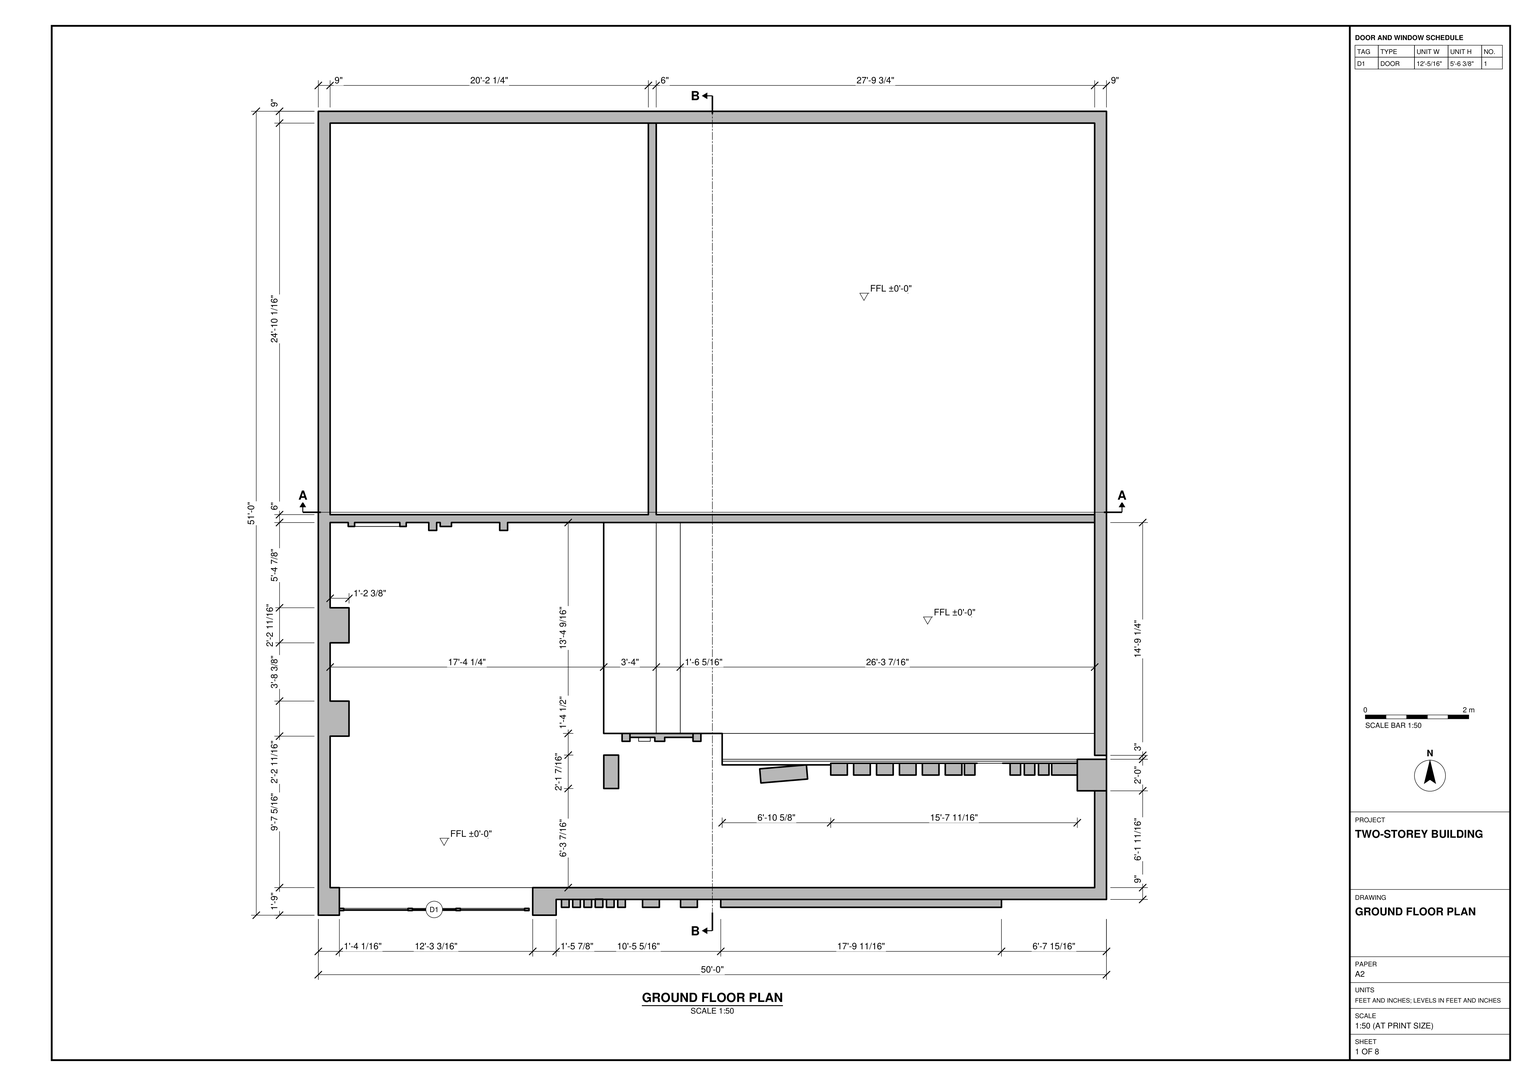
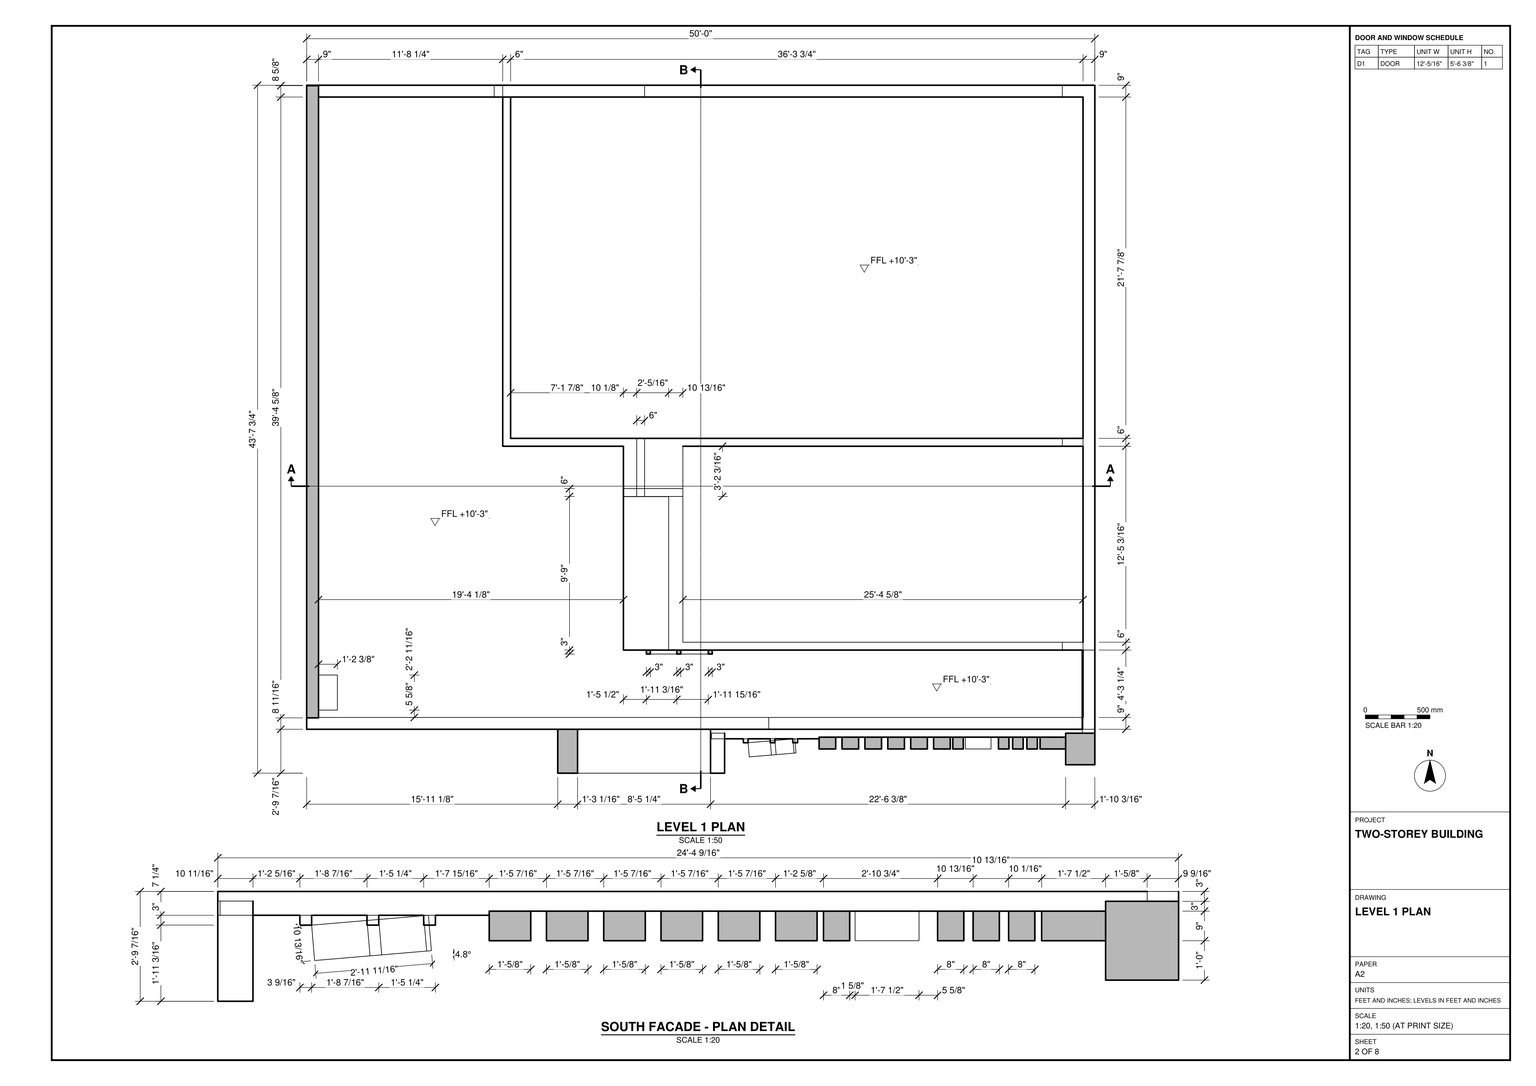
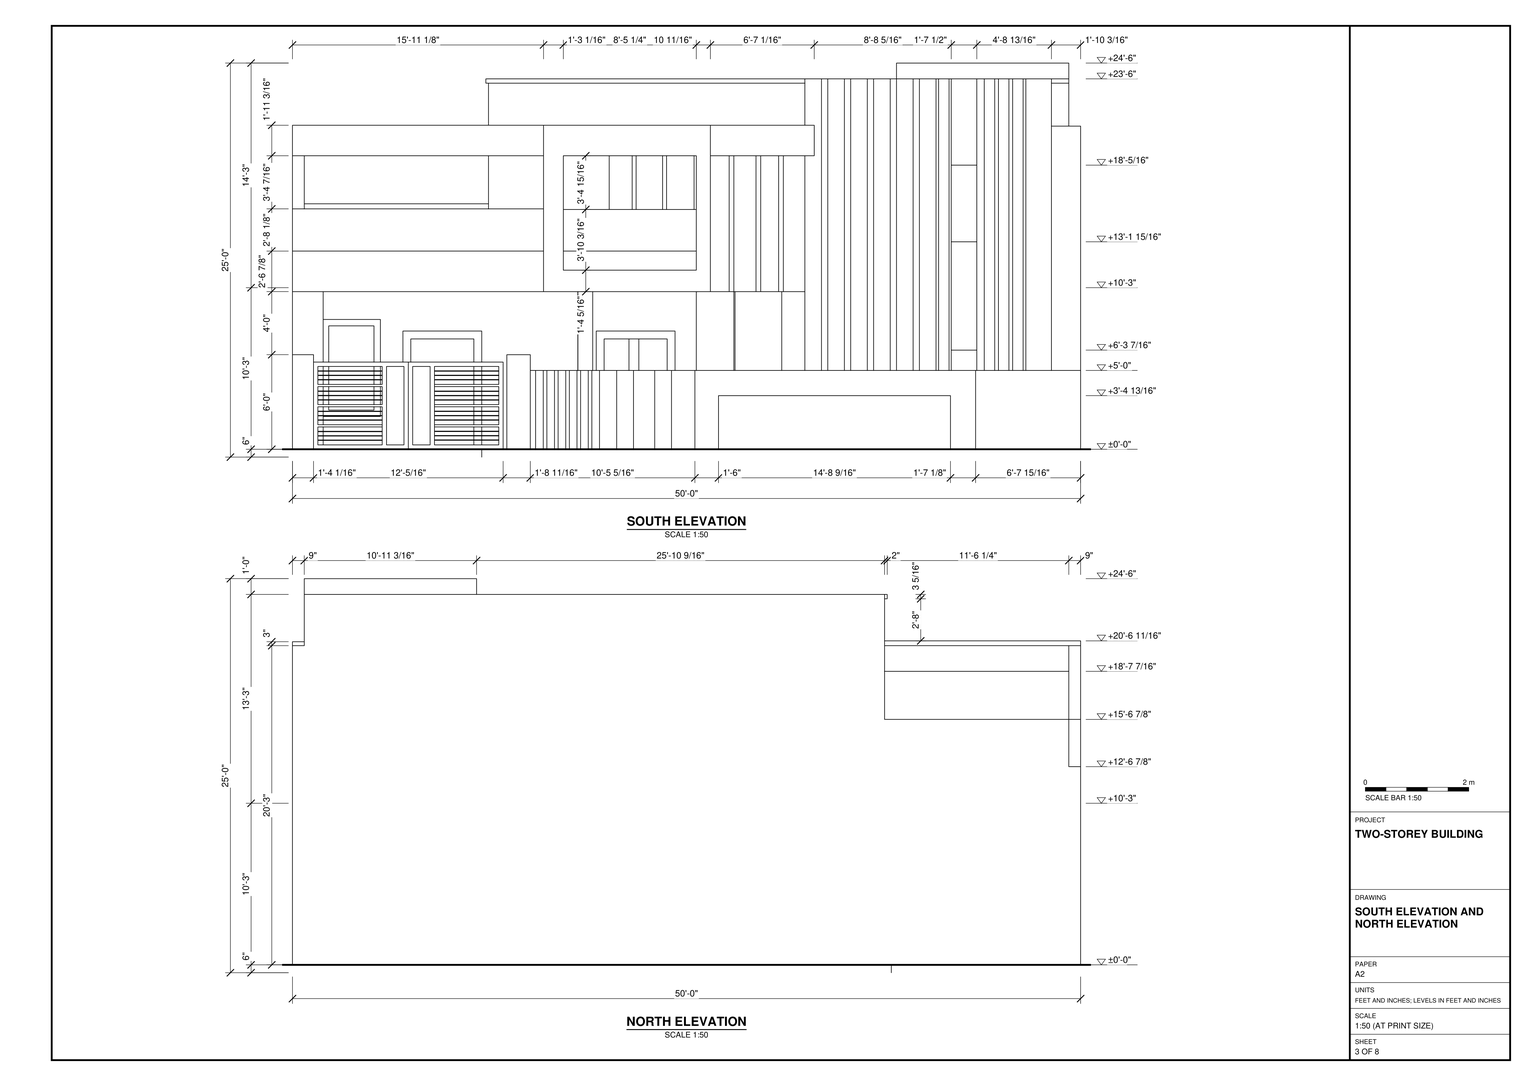
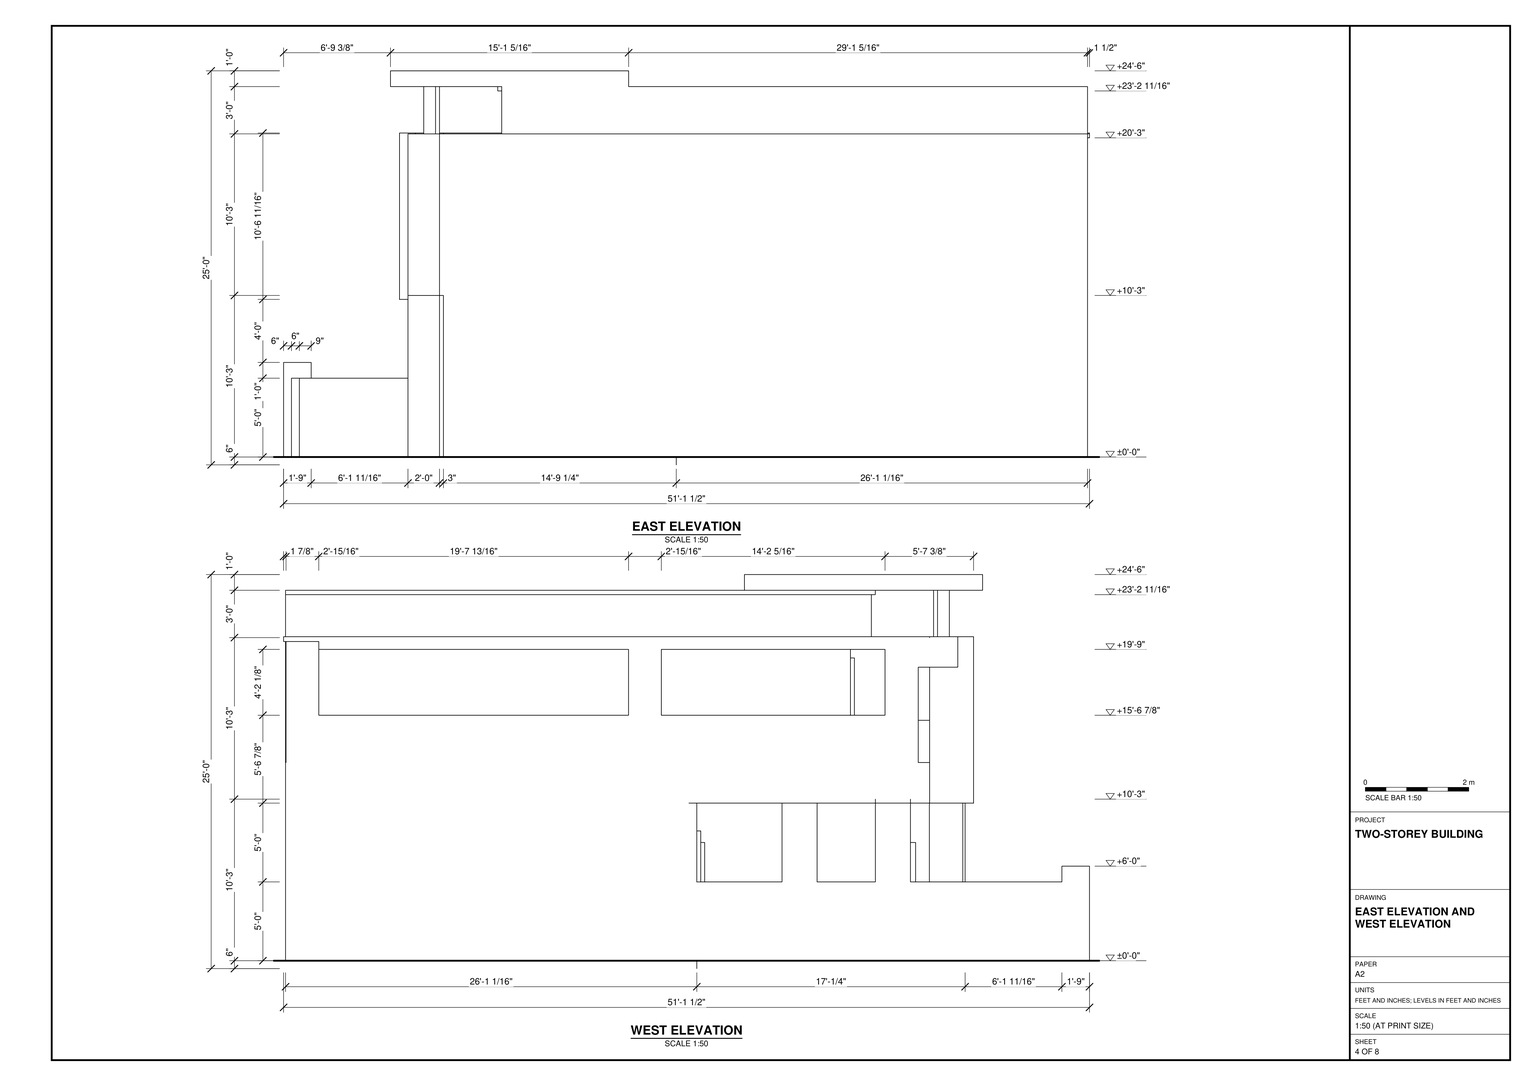
Build the two-storey building in SketchUp using task_files/diagram_01.pdf. Work in feet and inches. Set the overall width to 50'-0", the overall depth to 51'-1 1/2", and the overall height to 24'-6". Use ±0'-0" for the ground floor and +10'-3" for the upper floor.

Lay out each floor from its own plan. Use the 9" perimeter walls and 6" partitions where dimensioned. On the ground floor, divide the rear portion into two unequal bays and retain the open space behind the front gate. On the upper floor, follow the offsets in the partition layout rather than copying the walls below. Model the floor slabs, flat roof sections and changes in roof height to match the sections and elevations.

Place the slatted gate between posts at the left of the south frontage. Use the south elevation for the framed openings and horizontal bands, and the façade plan detail for the spacing and projection of the tall vertical fins on the right. Include the rectangular panel in the low front wall. Keep walls, slabs and roof sections in separate groups or components, group each furniture or joinery piece separately, and use components for repeated parts. Any decor or loose items shown may be represented by suitable library components. Save one SketchUp model as output_files/two_storey_building_with_screened_south_facade.skp.

# SketchUp Ruby script. Lengths in inches.
U = 1.inch
M = Sketchup.active_model
def pt(a) = Geom::Point3d.new(a.map { |v| v * U })
def face(e, loops, mat)
  f = e.add_face(loops[0].map { |a| pt(a) })
  loops[1..].each { |l| e.add_face(l.map { |a| pt(a) }).erase! }
  f.material = f.back_material = mat if mat
  f
end
# faces: each face lists its corners as indices into pts; further lists are holes
def faces(e, pts, list, mat = nil) = list.each { |f| face(e, (f[0].is_a?(Array) ? f : [f]).map { |l| l.map { |i| pts[i] } }, mat) }
# xy, xz, yz: faces in a plane at the given z, y or x. An outline is a flat list of corners, or four numbers for a rectangle; further outlines are holes
def ring(l) = l.size == 4 ? [[l[0], l[1]], [l[2], l[1]], [l[2], l[3]], [l[0], l[3]]] : l.each_slice(2).to_a
def flat(e, list, mat, &to3) = list.each { |f| face(e, (f[0].is_a?(Array) ? f : [f]).map { |l| ring(l).map { |u, v| to3.(u, v) } }, mat) }
def xy(e, z, list, mat = nil) = flat(e, list, mat) { |x, y| [x, y, z] }
def xz(e, y, list, mat = nil) = flat(e, list, mat) { |x, z| [x, y, z] }
def yz(e, x, list, mat = nil) = flat(e, list, mat) { |y, z| [x, y, z] }
def lines(e, pts, list) = list.each { |a, b| e.add_line(pt(pts[a]), pt(pts[b])) }
# prism: a flat outline (further loops are holes) pulled along v
def prism(e, loops, v, mat = nil)
  f = face(e, loops, mat); d = Geom::Vector3d.new(v.map { |x| x * U })
  f.pushpull(f.normal.samedirection?(d) ? d.length : -d.length)
end
def box(e, o, s, mat = nil) = prism(e, [[o, [o[0] + s[0], o[1], o[2]], [o[0] + s[0], o[1] + s[1], o[2]], [o[0], o[1] + s[1], o[2]]]], [0, 0, s[2]], mat)
def at(x, y, z, deg = 0) = Geom::Transformation.translation(pt([x, y, z])) * Geom::Transformation.rotation(ORIGIN, Z_AXIS, deg.degrees)
def axes(o, x, y, z) = Geom::Transformation.new([*x, 0, *y, 0, *z, 0, *pt(o).to_a, 1])
def part(name) = M.definitions.add(name)
# library, detail: a bought-in or finely detailed component or shape, given as its bounding box
def library(name, o, s) = part(name).tap { |d| box(d.entities, o, s) }
def detail(e, o, s) = box(e.add_group.entities, o, s)
def put(e, d, t, mat = nil) = e.add_instance(d, t).tap { |i| i.material = mat if mat }
def group(e, t, mat = nil) = e.add_group.tap { |g| g.transformation = t; g.material = mat if mat }.entities
root = M.entities
M.materials.add("[0035_Tan]").color = [155, 133, 103]
M.materials.add("[0042_Sienna]").color = [145, 74, 40]
M.materials.add("[0042_Sienna]1").color = [160, 82, 45]
M.materials.add("[0135_DarkGray]").color = [81, 81, 81]
M.materials.add("[Color C08]").color = [63, 31, 0]
M.materials.add("[Color C08]1").color = [61, 30, 0]
M.materials.add("[Formica Graystone]").color = [149, 146, 135]
M.materials.add("[Granite Brown]").color = [81, 67, 58]
M.materials.add("[Granite Dark Gray]").color = [69, 68, 68]
M.materials.add("[Sandstone]").color = [118, 81, 52]
M.materials.add("[Tile Mosaic Multi]").color = [135, 103, 96]
M.materials.add("[Translucent Glass Blue]").color = [100, 149, 237]
M.materials["[Translucent Glass Blue]"].alpha = 0.5
M.materials.add("[Wood Square Tile 01]").color = [164, 91, 44]
M.materials.add("[Wood Veneer 01]").color = [120, 70, 37]
c1 = library("gate (1)",[0,0,0],[171.26,1.97,78.74])
xy(root,0,[[0,0,16.04,12],[163.22,0,181.0625,12],[185.11,6,190.93,12],[193.67,6,199.49,12],[202.24,6,208.05,12],
  [210.8,6,216.61,12],[219.36,6,225.18,12],[227.92,6,233.74,12],[246.83,6,259.625,12],[275.77,6,288.5625,12],
  [0,12,0,136.3,9,136.3,9,21,16.04,21,16.04,12],[163.22,12,163.22,21,591,21,591,12,216.61,12,216.61,12.25,210.8,12.25,210.8,12],[210.8,12,216.61,12.25],[591,12,600,94.6875],[577.78,94.6875,591,118.6875],
  [591,94.6875,600,118.6875],[217.33,96.45,228.58,121.89],[390.09,106.6875,402.74,115.6875],[407.52,106.6875,420.18,115.6875],[424.96,106.6875,437.61,115.6875],
  [442.4,106.6875,455.05,115.6875],[459.84,106.6875,472.49,115.6875],[477.27,106.6875,489.93,115.6875],[491.875,106.6875,499.86,115.6875],[526.625,106.6875,534.61,115.6875],
  [537.4375,106.6875,545.42,115.6875],[548.25,106.6875,556.23,115.6875],[558.31,106.6875,577.78,115.6875],[307.4375,114.4375,390.09,114.4375,390.09,115.6875,577.78,115.6875,577.78,117.25,307.4375,117.25],[307.4375,117.25,577.78,118.6875],
  [307.4375,118.6875,600,118.6875,600,121.6875,591,121.6875,591,138.375,307.4375,138.375],[591,121.6875,591,603,9,603,9,304.9375,251.25,304.9375,251.25,603,257.25,603,257.25,304.9375,591,304.9375,591,298.9375,0,298.9375,0,612,600,612,600,121.6875],[231.25,132.375,237.25,138.375],[256.18,132.375,257.25,132.375,257.25,138.375,237.25,138.375,237.25,135.375,256.18,135.375],[257.25,132.375,263.69,132.375,263.69,135.375,275.5625,135.375,275.5625,138.375,257.25,138.375],
  [285.25,132.375,291.25,138.375],[275.5625,135.375,285.25,138.375],[0,136.3,23.375,162.99],[217.25,138.375,257.25,298.9375],[257.25,138.375,275.5625,298.9375],
  [275.5625,138.375,591,298.9375],[0,162.99,9,207.36],[0,207.36,23.375,234.05],[0,234.05,9,298.9375],[84.1,292.9375,90.1,298.9375],
  [138.1,292.9375,144.1,298.9375],[9,304.9375,251.25,603],[257.25,304.9375,591,603]])
xy(root,0,[[306.36,6,324.34,12],[500.93,6,520.07,12]],"[0135_DarkGray]")
xy(root,0,[[[9,21,591,21,591,94.6875,577.78,94.6875,577.78,106.6875,558.31,106.6875,558.31,115.6875,556.23,115.6875,556.23,106.6875,548.25,106.6875,548.25,115.6875,545.42,115.6875,545.42,106.6875,537.4375,106.6875,537.4375,115.6875,534.61,115.6875,534.61,106.6875,526.625,106.6875,526.625,115.6875,499.86,115.6875,499.86,106.6875,491.875,106.6875,491.875,115.6875,489.93,115.6875,489.93,106.6875,477.27,106.6875,477.27,115.6875,472.49,115.6875,472.49,106.6875,459.84,106.6875,459.84,115.6875,455.05,115.6875,455.05,106.6875,442.4,106.6875,442.4,115.6875,437.61,115.6875,437.61,106.6875,424.96,106.6875,424.96,115.6875,420.18,115.6875,420.18,106.6875,407.52,106.6875,407.52,115.6875,402.74,115.6875,402.74,106.6875,390.09,106.6875,390.09,114.4375,307.4375,114.4375,307.4375,138.375,291.25,138.375,291.25,132.375,285.25,132.375,285.25,135.375,263.69,135.375,263.69,132.375,256.18,132.375,256.18,135.375,237.25,135.375,237.25,132.375,231.25,132.375,231.25,138.375,217.25,138.375,217.25,298.9375,144.1,298.9375,144.1,292.9375,138.1,292.9375,138.1,298.9375,90.1,298.9375,90.1,292.9375,84.1,292.9375,84.1,298.9375,9,298.9375,9,234.05,23.375,234.05,23.375,207.36,9,207.36,9,162.99,23.375,162.99,23.375,136.3,9,136.3],[217.33,96.45,228.58,121.89]]],"[Wood Square Tile 01]")
xy(root,16.24,[[336.92,100.66,336.01,111.4375,371.57,114.4375,372.48,103.66]])
xy(root,24.96,[[22.76,295.9375,66.9375,298.9375]],"[Granite Dark Gray]")
xy(root,29.83,[[27.63,295.9375,62.07,298.9375]],"[Granite Dark Gray]")
xy(root,40.81,[[324.34,6,500.93,12]],"[0135_DarkGray]")
xy(root,60,[[181.0625,12,210.8,12,210.8,12.25,216.61,12.25,216.61,12,600,12,600,94.6875,591,94.6875,591,21,181.0625,21],[210.8,12,216.61,12.25],[0,21,9,136.3],[0,162.99,9,207.36],[0,234.05,9,298.9375]])
xy(root,60,[[185.11,6,190.93,12],[193.67,6,199.49,12],[202.24,6,208.05,12],[210.8,6,216.61,12],[219.36,6,225.18,12],
  [227.92,6,233.74,12]],"[0042_Sienna]1")
xy(root,60,[[246.83,6,259.625,12],[275.77,6,288.5625,12],[306.36,6,520.07,12]],"[0135_DarkGray]")
xy(root,72,[[0,0,16.04,21],[163.22,0,181.0625,21]])
xy(root,75.46,[[501.49,106.6875,520.97,115.6875]])
xy(root,84,[[256.18,132.375,256.18,135.375,237.25,135.375,237.25,138.375,285.25,138.375,285.25,135.375,263.69,135.375,263.69,132.375]])
xy(root,84,[[237.25,132.375,256.18,135.375],[263.69,132.375,285.25,135.375],[90.1,292.9375,138.1,298.9375]],"[Sandstone]")
xy(root,90,[[231.25,132.375,291.25,138.375],[84.1,292.9375,144.1,298.9375]],"[Sandstone]")
xy(root,93.95,[[27.63,295.9375,62.07,298.9375]],"[Granite Dark Gray]")
xy(root,98.82,[[22.76,295.9375,66.9375,298.9375]],"[Granite Dark Gray]")
xy(root,120,[[332.4375,111.4375,336.01,114.4375],[336.01,111.4375,336.01,114.4375,352.875,114.4375,352.875,112.86],[352.875,111.4375,352.875,112.86,353,111.4375],[353,111.4375,352.875,112.86,356.45,113.16,356.45,111.4375],[370.125,111.4375,370.125,114.32,370.37,111.4375],
  [370.37,111.4375,370.125,114.32,371.57,114.4375,371.82,111.4375],[371.82,111.4375,371.57,114.4375,373.7,114.4375,373.7,111.4375],[352.875,112.86,352.875,114.4375,356.45,114.4375,356.45,113.16],[356.45,113.16,356.45,114.4375,370.125,114.4375,370.125,114.32],[370.125,114.32,370.125,114.4375,371.57,114.4375],
  [307.4375,114.4375,308.13,118.75],[308.13,114.4375,318.15,118.75],[307.4375,121.6875,575.24,138.375],[575.24,121.6875,591,138.375],[217.25,138.375,275.5625,298.8125],
  [275.5625,138.375,575.24,298.9375],[575.24,138.375,591,298.9375],[9,298.8125,217.25,298.9375],[217.25,298.8125,275.5625,298.9375],[0,298.9375,9,304.9375],
  [9,298.9375,251.25,304.9375],[251.25,298.9375,257.25,304.9375],[257.25,298.9375,575.24,304.9375],[575.24,298.9375,591,304.9375],[9,304.9375,251.25,603],
  [251.25,304.9375,257.25,603],[257.25,304.9375,575.24,603],[575.24,304.9375,591,603]])
xy(root,120,[[0,121.6875,0,207.36,23.375,207.36,23.375,234.05,0,234.05,0,298.9375,9,298.9375,9,298.8125,217.25,298.8125,217.25,121.6875]],"[0035_Tan]")
xy(root,120,[[191.13,88.25,191.13,121.6875,217.25,121.6875,217.25,138.375,307.4375,138.375,307.4375,114.4375,318.15,114.4375,318.15,88.25]],"[0135_DarkGray]")
xy(root,120,[[336.92,100.66,353.78,102.09,353,111.4375,352.875,111.4375,352.875,112.86,336.01,111.4375],[353.78,102.09,357.36,102.39,356.45,113.16,356.45,111.4375,353,111.4375],[357.36,102.39,371.03,103.54,370.37,111.4375,370.125,111.4375,370.125,114.32,356.45,113.16],[371.03,103.54,372.48,103.66,371.82,111.4375,370.37,111.4375]],"[Granite Brown]")
xy(root,122.4375,[[217.33,96.45,228.58,121.89]])
xy(root,123,[[351.77,121.6875,590.4375,130.6875],[590.4375,121.6875,591,130.6875],[590.4375,130.6875,591,181.97],[9,136.3,23.375,162.99],[286.375,187.97,591,337.16],
  [155.25,343.16,591,603]])
xy(root,123,[[9,130.6875,590.4375,130.6875,590.4375,181.97,241.125,181.97,241.125,337.16,149.25,337.16,149.25,603,9,603,9,162.99,23.375,162.99,23.375,136.3,9,136.3]],"[Tile Mosaic Multi]")
xy(root,136.34,[[206.21,88.25,307.4375,121.6875]],"[0135_DarkGray]")
xy(root,150.875,[[0,121.6875,351.77,121.6875,351.77,130.6875,9,130.6875,9,130.375,0,130.375]])
xy(root,157.94,[[501.49,106.6875,520.97,115.6875]],"[Color C08]")
xy(root,161.89,[[258.61,178.97,308.74,181.97]],"[Granite Dark Gray]")
xy(root,164.89,[[261.61,178.97,281.79,181.97],[284.79,178.97,305.74,181.97]],"[Granite Dark Gray]")
xy(root,186.875,[[0,155.65,9,325.9375],[0,350.9,9,586.6875],[9,603,149.25,603,149.25,612,0,612,0,611.65,9,611.65]])
xy(root,216.3,[[501.49,106.6875,520.97,115.6875]],"[Color C08]")
xy(root,223.45,[[0,100.25,191.13,130.375],[191.13,100.25,206.21,114.4375],[307.4375,100.25,318.15,114.4375],[318.15,100.25,318.15,114.4375,332.4375,114.4375,332.4375,111.4375,336.01,111.4375,336.01,114.4375,352.875,114.4375,352.875,111.4375,356.45,111.4375,356.45,114.4375,370.125,114.4375,370.125,111.4375,373.7,111.4375,373.7,114.4375,390.09,114.4375,390.09,106.6875,397.21,106.6875,397.21,100.25],[332.4375,111.4375,332.4375,114.4375,318.15,114.4375,318.15,115.6875,370.125,115.6875,370.125,114.4375,356.45,114.4375,356.45,111.4375,352.875,111.4375,352.875,114.4375,336.01,114.4375,336.01,111.4375],
  [370.125,111.4375,370.125,115.6875,390.09,115.6875,390.09,114.4375,373.7,114.4375,373.7,111.4375],[191.13,114.4375,206.21,118.75],[307.4375,114.4375,318.15,115.6875],[307.4375,115.6875,318.15,116.375],[191.13,118.75,206.21,121.6875],
  [191.13,121.6875,206.21,130.375]])
xy(root,223.45,[[206.21,88.25,307.4375,130.375]],"[0135_DarkGray]")
xy(root,227.51,[[261.61,178.97,281.79,181.97],[284.79,178.97,305.74,181.97]],"[Granite Dark Gray]")
xy(root,230.51,[[258.61,178.97,308.74,181.97]])
xy(root,232.39,[[307.4375,115.6875,370.125,117.25],[307.4375,117.25,370.125,118.6875],[307.4375,118.6875,370.125,121.6875],[307.4375,121.6875,370.125,130.375]])
xy(root,237,[[0,155.65,9,325.9375],[0,350.9,9,586.6875]])
xy(root,243,[[149.25,121.6875,370.125,130.375],[370.125,121.6875,370.125,130.375,149.25,130.375,149.25,337.16,241.125,337.16,241.125,181.97,590.4375,181.97,590.4375,121.6875],[590.4375,121.6875,591,181.97],[[9,130.375,9,603,18.125,603,18.125,580.6,132.125,580.6,132.125,603,149.25,603,149.25,130.375],[18.125,373.23,132.125,396.54],[18.125,262.04,132.125,285.35],[18.125,187.92,132.125,211.23],[18.125,299.1,132.125,322.42],[18.125,521.48,132.125,544.79],[18.125,224.98,132.125,248.29],[18.125,447.35,132.125,470.67],[18.125,336.17,132.125,359.48],[18.125,551.67,132.125,574.98],[18.125,484.42,132.125,507.73],[18.125,410.29,132.125,433.6],[18.125,150.85,132.125,174.17]],[241.125,181.97,280.375,187.97],
  [280.375,181.97,286.375,187.97],[286.375,181.97,286.375,187.97,280.375,187.97,280.375,337.16,591,337.16,591,181.97],[241.125,187.97,280.375,337.16],[149.25,337.16,286.375,343.16],[286.375,337.16,591,343.16],
  [149.25,343.16,155.25,603],[155.25,343.16,286.375,603],[286.375,343.16,591,603],[0,586.6875,9,603],[0,603,9,611.65],
  [9,603,9,611.65,0,611.65,0,613.5,149.25,613.5,149.25,603,132.125,603,132.125,603.92,18.125,603.92,18.125,603],[18.125,603,132.125,603.92]])
xy(root,246,[[577.78,94.6875,600,118.6875],[370.125,117.25,577.78,118.6875],[370.125,118.6875,591,118.6875,591,166.06,149.25,166.06,149.25,121.6875,370.125,121.6875],[591,118.6875,600,612],[149.25,166.06,591,207.93]])
xy(root,246.66,[[0,100.25,191.13,100.25,191.13,118.75,318.15,118.75,318.15,100.25,397.21,100.25,397.21,106.6875,390.09,106.6875,390.09,115.6875,370.125,115.6875,370.125,121.6875,0,121.6875],[191.13,100.25,318.15,114.4375],[191.13,114.4375,318.15,118.75],[370.125,115.6875,390.09,118.6875],[[0,121.6875,149.25,613.5],[18.125,373.23,132.125,396.54],[18.125,187.92,132.125,211.23],[18.125,224.98,132.125,248.29],[18.125,262.04,132.125,285.35],[18.125,299.1,132.125,322.42],[18.125,336.17,132.125,359.48],[18.125,410.29,132.125,433.6],[18.125,447.35,132.125,470.67],[18.125,484.42,132.125,507.73],[18.125,521.48,132.125,544.79],[18.125,551.67,132.125,574.98],[18.125,580.6,132.125,603.92],[18.125,150.85,132.125,174.17]]])
xy(root,246.66,[[191.13,88.25,318.15,100.25]],"[0135_DarkGray]")
xy(root,278.69,[[147.25,163.06,147.25,612,149.25,612,149.25,166.06,591,166.06,591,163.06]])
xy(root,282,[[459.84,81.375,459.84,106.6875,472.49,106.6875,472.49,115.6875,477.27,115.6875,477.27,106.6875,489.93,106.6875,489.93,115.6875,491.875,115.6875,491.875,106.6875,499.86,106.6875,499.86,115.6875,501.49,115.6875,501.49,106.6875,520.97,106.6875,520.97,115.6875,526.625,115.6875,526.625,106.6875,534.61,106.6875,534.61,115.6875,537.4375,115.6875,537.4375,106.6875,545.42,106.6875,545.42,115.6875,548.25,115.6875,548.25,106.6875,556.23,106.6875,556.23,115.6875,558.31,115.6875,558.31,106.6875,577.78,106.6875,577.78,118.6875,459.84,118.6875,459.84,161.75,591,161.75,591,81.375],[459.84,106.6875,472.49,115.6875],[477.27,106.6875,489.93,115.6875],[491.875,106.6875,499.86,115.6875],[501.49,106.6875,520.97,115.6875],
  [526.625,106.6875,534.61,115.6875],[537.4375,106.6875,545.42,115.6875],[548.25,106.6875,556.23,115.6875],[558.31,106.6875,577.78,115.6875],[390.09,115.6875,459.84,118.6875],
  [459.84,115.6875,577.78,118.6875],[459.84,161.75,591,163.06],[147.25,163.06,459.84,163.06,459.84,166.06,149.25,166.06,149.25,612,147.25,612],[459.84,163.06,591,166.06],[149.25,166.06,459.84,166.06,459.84,262.67,591,262.67,591,612,149.25,612]])
xy(root,282,[[390.09,106.6875,402.74,115.6875],[407.52,106.6875,420.18,115.6875],[424.96,106.6875,437.61,115.6875],[442.4,106.6875,455.05,115.6875]],"[Color C08]1")
xy(root,294,[[459.84,81.375,591,262.67]])
xz(root,0,[[0,0,16.04,72],[163.22,0,181.0625,72]])
xz(root,6,[[185.11,0,190.93,60],[193.67,0,199.49,60],[202.24,0,208.05,60],[210.8,0,216.61,60],[219.36,0,225.18,60],
  [227.92,0,233.74,60]],"[0042_Sienna]1")
xz(root,6,[[246.83,0,259.625,60],[275.77,0,288.5625,60],[306.36,0,324.34,0,324.34,40.81,500.93,40.81,500.93,0,520.07,0,520.07,60,306.36,60]],"[0135_DarkGray]")
xz(root,12,[[181.0625,0,185.11,60],[185.11,0,190.93,60],[190.93,0,193.67,60],[193.67,0,199.49,60],[199.49,0,202.24,60],
  [202.24,0,208.05,60],[208.05,0,210.8,60],[210.8,0,216.61,60],[216.61,0,219.36,60],[219.36,0,225.18,60],
  [225.18,0,227.92,60],[227.92,0,233.74,60],[233.74,0,246.83,60],[246.83,0,259.625,60],[259.625,0,275.77,60],
  [275.77,0,288.5625,60],[306.36,0,306.36,60,520.07,60,520.07,0,500.93,0,500.93,40.81,324.34,40.81,324.34,0],[520.07,0,600,60]])
xz(root,12,[[288.5625,0,306.36,60]],"[0135_DarkGray]")
xz(root,12,[[324.34,0,500.93,40.81]],"[Formica Graystone]")
xz(root,12.25,[[210.8,0,216.61,60]])
xz(root,21,[[9,0,16.04,60],[163.22,0,591,60],[0,60,9,72],[9,60,16.04,72],[163.22,60,181.0625,72]])
xz(root,81.375,[[459.84,282,591,294]])
xz(root,88.25,[[[191.13,120,318.15,246.66],[206.21,136.34,307.4375,223.45]]],"[0135_DarkGray]")
xz(root,94.6875,[[577.78,0,591,0,591,60,600,60,600,246,577.78,246],[591,0,600,60]])
xz(root,96.45,[[217.33,0,228.58,122.4375]],"[0135_DarkGray]")
xz(root,100.25,[[0,223.45,191.13,246.66],[318.15,223.45,397.21,246.66]])
xz(root,106.6875,[[390.09,223.45,397.21,246.66]])
xz(root,106.6875,[[491.875,0,499.86,282],[526.625,0,534.61,282],[537.4375,0,545.42,282],[548.25,0,556.23,282]],"[0042_Sienna]")
xz(root,106.6875,[[390.09,0,402.74,0,402.74,282,390.09,282,390.09,246.66,397.21,246.66,397.21,223.45,390.09,223.45],[407.52,0,420.18,282],[424.96,0,437.61,282],[442.4,0,455.05,282],[459.84,0,472.49,282],
  [477.27,0,489.93,282],[501.49,75.46,520.97,157.94],[501.49,216.3,520.97,282]],"[Color C08]")
xz(root,106.6875,[[558.31,0,577.78,282]],"[Color C08]1")
xz(root,111.4375,[[332.4375,120,336.01,223.45],[352.875,120,356.45,223.45],[370.125,120,373.7,223.45]])
xz(root,114.4375,[[307.4375,0,390.09,120]],"[0035_Tan]")
xz(root,114.4375,[[318.15,120,332.4375,223.45],[336.01,120,352.875,223.45],[356.45,120,370.125,223.45],[373.7,120,390.09,223.45]],"[Wood Veneer 01]")
xz(root,115.6875,[[390.09,0,402.74,282],[407.52,0,420.18,282],[424.96,0,437.61,282],[442.4,0,455.05,282],[459.84,0,472.49,282],
  [477.27,0,489.93,282],[489.93,0,491.875,282],[491.875,0,499.86,282],[499.86,0,501.49,282],[520.97,0,526.625,282],
  [526.625,0,534.61,282],[534.61,0,537.4375,282],[537.4375,0,545.42,282],[545.42,0,548.25,282],[548.25,0,556.23,282],
  [556.23,0,558.31,282],[558.31,0,577.78,282],[501.49,75.46,520.97,157.94],[501.49,216.3,520.97,282],[307.4375,223.45,370.125,232.39],
  [370.125,223.45,390.09,246.66]])
xz(root,115.6875,[[402.74,0,407.52,282],[420.18,0,424.96,282],[437.61,0,442.4,282],[455.05,0,459.84,282],[472.49,0,477.27,282],
  [501.49,157.94,520.97,216.3]],"[Color C08]")
xz(root,118.6875,[[577.78,0,600,246],[370.125,246,370.125,246.66,390.09,246.66,390.09,282,577.78,282,577.78,246]])
xz(root,121.6875,[[591,0,600,120],[0,120,191.13,150.875],[191.13,123,191.13,136.34,307.4375,136.34,307.4375,150.875,351.77,150.875,351.77,123],[351.77,123,351.77,150.875,307.4375,150.875,307.4375,232.39,370.125,232.39,370.125,243,590.4375,243,590.4375,123],[191.13,136.34,206.21,150.875],
  [206.21,136.34,307.4375,150.875],[191.13,150.875,206.21,223.45],[149.25,243,370.125,246],[0,246,149.25,246.66]])
xz(root,121.6875,[[0,150.875,191.13,183.01],[206.21,150.875,307.4375,182.54]],"[Translucent Glass Blue]")
xz(root,121.89,[[217.33,0,228.58,122.4375]],"[0135_DarkGray]")
xz(root,130.375,[[0,150.875,9,223.45],[9,223.45,9,243,370.125,243,370.125,232.39,307.4375,232.39,307.4375,223.45]])
xz(root,130.6875,[[9,123,351.77,150.875]])
xz(root,132.375,[[231.25,0,237.25,0,237.25,84,285.25,84,285.25,0,291.25,0,291.25,90,231.25,90],[256.18,0,263.69,84],[248.27,36.05,249.42,36.2,250.49,36.64,251.41,37.35,252.12,38.27,252.56,39.34,252.71,40.49,252.56,41.64,252.12,42.71,251.41,43.625,250.49,44.33,249.42,44.77,248.27,44.93,247.125,44.77,246.05,44.33,245.13,43.625,244.43,42.71,243.99,41.64,243.84,40.49,243.99,39.34,244.43,38.27,245.13,37.35,246.05,36.64,247.125,36.2]],"[Sandstone]")
xz(root,135.375,[[[237.25,0,256.18,84],[248.27,36.05,247.125,36.2,246.05,36.64,245.13,37.35,244.43,38.27,243.99,39.34,243.84,40.49,243.99,41.64,244.43,42.71,245.13,43.625,246.05,44.33,247.125,44.77,248.27,44.93,249.42,44.77,250.49,44.33,251.41,43.625,252.12,42.71,252.56,41.64,252.71,40.49,252.56,39.34,252.12,38.27,251.41,37.35,250.49,36.64,249.42,36.2]],[263.69,0,285.25,84]],"[Sandstone]")
xz(root,136.3,[[9,0,23.375,0,23.375,123,0,123,0,60,9,60]],"[0135_DarkGray]")
xz(root,138.375,[[231.25,0,231.25,90,291.25,90,291.25,0,285.25,0,285.25,84,237.25,84,237.25,0],[237.25,0,285.25,84]])
xz(root,138.375,[[217.25,0,231.25,0,231.25,90,291.25,90,291.25,0,307.4375,0,307.4375,120,217.25,120]],"[0035_Tan]")
xz(root,150.85,[[18.125,243,132.125,246.66]])
xz(root,155.65,[[0,186.875,9,237]])
xz(root,162.99,[[9,0,9,60,0,60,0,123,23.375,123,23.375,0]],"[0135_DarkGray]")
xz(root,163.06,[[147.25,278.69,591,282]])
xz(root,166.06,[[149.25,278.69,591,282]])
xz(root,166.06,[[149.25,246,591,278.69]],"[0135_DarkGray]")
xz(root,174.17,[[18.125,243,132.125,246.66]])
xz(root,178.97,[[[258.61,161.89,308.74,230.51],[284.79,164.89,305.74,227.51],[261.61,164.89,281.79,227.51]]],"[Granite Dark Gray]")
xz(root,181.97,[[590.4375,123,591,243],[[258.61,161.89,308.74,230.51],[284.79,164.89,305.74,227.51],[261.61,164.89,281.79,227.51]],[280.375,243,286.375,243.125],[286.375,243,588.125,243.125],[588.125,243,591,243.125]])
xz(root,181.97,[[[241.125,123,590.4375,243],[258.61,161.89,308.74,230.51]]],"[Formica Graystone]")
xz(root,181.97,[[261.61,164.89,281.79,227.51],[284.79,164.89,305.74,227.51]],"[Translucent Glass Blue]")
xz(root,187.92,[[18.125,243,132.125,246.66]])
xz(root,207.36,[[9,0,23.375,0,23.375,120,0,120,0,60,9,60]],"[0135_DarkGray]")
xz(root,211.23,[[18.125,243,132.125,246.66]])
xz(root,224.98,[[18.125,243,132.125,246.66]])
xz(root,234.05,[[9,0,9,60,0,60,0,120,23.375,120,23.375,0]],"[0135_DarkGray]")
xz(root,248.29,[[18.125,243,132.125,246.66]])
xz(root,262.04,[[18.125,243,132.125,246.66]])
xz(root,262.67,[[459.84,282,591,294]])
xz(root,285.35,[[18.125,243,132.125,246.66]])
xz(root,292.9375,[[84.1,0,90.1,0,90.1,84,138.1,84,138.1,0,144.1,0,144.1,90,84.1,90]],"[Sandstone]")
xz(root,295.9375,[[[22.76,24.96,66.9375,98.82],[27.63,29.83,62.07,93.95]]],"[Granite Dark Gray]")
xz(root,295.9375,[[97.08,43.46,98.21,43.61,99.27,44.05,100.18,44.75,100.87,45.65,101.31,46.71,101.46,47.84,101.31,48.97,100.87,50.03,100.18,50.93,99.27,51.63,98.21,52.06,97.08,52.21,95.95,52.06,94.9,51.63,93.99,50.93,93.29,50.03,92.86,48.97,92.71,47.84,92.86,46.71,93.29,45.65,93.99,44.75,94.9,44.05,95.95,43.61]],"[Sandstone]")
xz(root,298.9375,[[217.25,0,257.25,120],[257.25,0,275.5625,120],[275.5625,0,591,120]])
xz(root,298.9375,[[[9,0,84.1,0,84.1,90,144.1,90,144.1,0,217.25,0,217.25,120,0,120,0,60,9,60],[22.76,24.96,66.9375,98.82]]],"[0035_Tan]")
xz(root,298.9375,[[[90.1,0,138.1,84],[97.08,43.46,95.95,43.61,94.9,44.05,93.99,44.75,93.29,45.65,92.86,46.71,92.71,47.84,92.86,48.97,93.29,50.03,93.99,50.93,94.9,51.63,95.95,52.06,97.08,52.21,98.21,52.06,99.27,51.63,100.18,50.93,100.87,50.03,101.31,48.97,101.46,47.84,101.31,46.71,100.87,45.65,100.18,44.75,99.27,44.05,98.21,43.61]]],"[Sandstone]")
xz(root,298.9375,[[27.63,29.83,62.07,93.95]],"[Translucent Glass Blue]")
xz(root,299.1,[[18.125,243,132.125,246.66]])
xz(root,304.9375,[[9,0,251.25,120],[257.25,0,591,120]])
xz(root,322.42,[[18.125,243,132.125,246.66]])
xz(root,325.9375,[[0,186.875,9,237]])
xz(root,336.17,[[18.125,243,132.125,246.66]])
xz(root,337.16,[[286.375,123,591,243],[149.25,243,280.375,243.125]])
xz(root,337.16,[[149.25,123,241.125,243]],"[Formica Graystone]")
xz(root,343.16,[[155.25,123,591,243]])
xz(root,350.9,[[0,186.875,9,237]])
xz(root,359.48,[[18.125,243,132.125,246.66]])
xz(root,373.23,[[18.125,243,132.125,246.66]])
xz(root,396.54,[[18.125,243,132.125,246.66]])
xz(root,410.29,[[18.125,243,132.125,246.66]])
xz(root,433.6,[[18.125,243,132.125,246.66]])
xz(root,447.35,[[18.125,243,132.125,246.66]])
xz(root,470.67,[[18.125,243,132.125,246.66]])
xz(root,484.42,[[18.125,243,132.125,246.66]])
xz(root,507.73,[[18.125,243,132.125,246.66]])
xz(root,521.48,[[18.125,243,132.125,246.66]])
xz(root,544.79,[[18.125,243,132.125,246.66]])
xz(root,551.67,[[18.125,243,132.125,246.66]])
xz(root,574.98,[[18.125,243,132.125,246.66]])
xz(root,580.6,[[18.125,243,132.125,246.66]])
xz(root,586.6875,[[0,186.875,9,237]])
xz(root,603,[[9,0,251.25,120],[251.25,0,257.25,120],[257.25,0,591,120],[142.75,120,251.25,123],[9,123,149.25,186.875],
  [149.25,123,155.25,243],[155.25,123,591,243]])
xz(root,603.92,[[18.125,243,132.125,246.66]])
xz(root,611.65,[[0,150.875,9,186.875],[0,186.875,9,243]])
xz(root,612,[[0,0,0,186.875,149.25,186.875,149.25,282,591,282,591,243,600,243,600,0],[591,243,600,246],[147.25,278.69,149.25,282]])
xz(root,613.5,[[0,243,149.25,246.66]])
yz(root,0,[[[0,0,0,72,21,72,21,60,136.3,60,136.3,120,162.99,120,162.99,60,207.36,60,207.36,120,234.05,120,234.05,60,298.9375,60,298.9375,120,121.6875,120,121.6875,150.875,130.375,150.875,130.375,223.45,100.25,223.45,100.25,246.66,613.5,246.66,613.5,243,611.65,243,611.65,150.875,612,150.875,612,0],[350.9,186.875,586.6875,237],[155.65,186.875,325.9375,237]],[611.65,150.875,612,186.875]])
yz(root,0,[[121.6875,150.875,130.375,183.01]],"[Translucent Glass Blue]")
yz(root,9,[[21,0,136.3,60],[162.99,0,207.36,60],[234.05,0,298.9375,60],[304.9375,0,603,120],[[130.6875,123,603,123,603,243,586.6875,243,586.6875,186.875,350.9,186.875,350.9,237,586.6875,237,586.6875,243,130.375,243,130.375,150.875,130.6875,150.875],[155.65,186.875,325.9375,237]],
  [603,150.875,611.65,186.875],[603,186.875,611.65,243]])
yz(root,16.04,[[0,0,21,72]])
yz(root,18.125,[[150.85,243,174.17,246.66],[187.92,243,211.23,246.66],[224.98,243,248.29,246.66],[262.04,243,285.35,246.66],[299.1,243,322.42,246.66],
  [336.17,243,359.48,246.66],[373.23,243,396.54,246.66],[410.29,243,433.6,246.66],[447.35,243,470.67,246.66],[484.42,243,507.73,246.66],
  [521.48,243,544.79,246.66],[551.67,243,574.98,246.66],[580.6,243,603.92,246.66]])
yz(root,22.76,[[295.9375,24.96,298.9375,98.82]],"[Granite Dark Gray]")
yz(root,23.375,[[207.36,0,234.05,120]])
yz(root,23.375,[[136.3,0,162.99,123]],"[0135_DarkGray]")
yz(root,27.63,[[295.9375,29.83,298.9375,93.95]],"[Granite Dark Gray]")
yz(root,62.07,[[295.9375,29.83,298.9375,93.95]],"[Granite Dark Gray]")
yz(root,66.9375,[[295.9375,24.96,298.9375,98.82]],"[Granite Dark Gray]")
yz(root,84.1,[[292.9375,0,298.9375,90]],"[Sandstone]")
yz(root,90.1,[[292.9375,0,298.9375,84]],"[Sandstone]")
yz(root,132.125,[[150.85,243,174.17,246.66],[187.92,243,211.23,246.66],[224.98,243,248.29,246.66],[262.04,243,285.35,246.66],[299.1,243,322.42,246.66],
  [336.17,243,359.48,246.66],[373.23,243,396.54,246.66],[410.29,243,433.6,246.66],[447.35,243,470.67,246.66],[484.42,243,507.73,246.66],
  [521.48,243,544.79,246.66],[551.67,243,574.98,246.66],[580.6,243,603.92,246.66]])
yz(root,138.1,[[292.9375,0,298.9375,84]],"[Sandstone]")
yz(root,144.1,[[292.9375,0,298.9375,90]],"[Sandstone]")
yz(root,147.25,[[163.06,278.69,612,282]])
yz(root,149.25,[[603,186.875,612,243],[121.6875,243,337.16,243.125],[337.16,243,612,243.125],[612,243,613.5,243.125],[121.6875,243.125,612,246],
  [612,243.125,613.5,246],[121.6875,246,166.06,246.66],[166.06,246,207.93,246.66],[207.93,246,612,246.66],[612,246,613.5,246.66],
  [166.06,278.69,612,282]])
yz(root,149.25,[[166.06,246.66,612,278.69]],"[0135_DarkGray]")
yz(root,149.25,[[337.16,123,603,243]],"[Formica Graystone]")
yz(root,155.25,[[343.16,123,603,243]])
yz(root,163.22,[[0,0,21,72]])
yz(root,181.0625,[[0,0,12,0,12,60,21,60,21,72,0,72]])
yz(root,185.11,[[6,0,12,60]],"[0042_Sienna]1")
yz(root,190.93,[[6,0,12,60]],"[0042_Sienna]1")
yz(root,191.13,[[100.25,223.45,114.4375,246.66],[114.4375,223.45,118.75,246.66]])
yz(root,191.13,[[88.25,120,88.25,246.66,100.25,246.66,100.25,223.45,121.6875,223.45,121.6875,120]],"[0135_DarkGray]")
yz(root,193.67,[[6,0,12,60]],"[0042_Sienna]1")
yz(root,199.49,[[6,0,12,60]],"[0042_Sienna]1")
yz(root,202.24,[[6,0,12,60]],"[0042_Sienna]1")
yz(root,206.21,[[88.25,136.34,121.6875,223.45]],"[0135_DarkGray]")
yz(root,208.05,[[6,0,12,60]],"[0042_Sienna]1")
yz(root,210.8,[[12,0,12.25,60]])
yz(root,210.8,[[6,0,12,60]],"[0042_Sienna]1")
yz(root,216.61,[[12,0,12.25,60]])
yz(root,216.61,[[6,0,12,60]],"[0042_Sienna]1")
yz(root,217.25,[[138.375,0,298.9375,120]],"[0035_Tan]")
yz(root,217.33,[[96.45,0,121.89,122.4375]],"[0135_DarkGray]")
yz(root,219.36,[[6,0,12,60]],"[0042_Sienna]1")
yz(root,225.18,[[6,0,12,60]],"[0042_Sienna]1")
yz(root,227.92,[[6,0,12,60]],"[0042_Sienna]1")
yz(root,228.58,[[96.45,0,121.89,122.4375]],"[0135_DarkGray]")
yz(root,231.25,[[132.375,0,138.375,90]],"[Sandstone]")
yz(root,233.74,[[6,0,12,60]],"[0042_Sienna]1")
yz(root,237.25,[[135.375,0,138.375,84]])
yz(root,237.25,[[132.375,0,135.375,84]],"[Sandstone]")
yz(root,241.125,[[181.97,123,337.16,243]],"[Formica Graystone]")
yz(root,246.83,[[6,0,12,60]],"[0135_DarkGray]")
yz(root,251.25,[[304.9375,0,603,120]])
yz(root,256.18,[[132.375,0,135.375,84]],"[Sandstone]")
yz(root,257.25,[[304.9375,0,603,120]])
yz(root,258.61,[[178.97,161.89,181.97,230.51]],"[Granite Dark Gray]")
yz(root,259.625,[[6,0,12,60]],"[0135_DarkGray]")
yz(root,261.61,[[178.97,164.89,181.97,227.51]],"[Granite Dark Gray]")
yz(root,263.69,[[132.375,0,135.375,84]],"[Sandstone]")
yz(root,275.77,[[6,0,12,60]],"[0135_DarkGray]")
yz(root,280.375,[[181.97,243,187.97,243.125],[187.97,243,337.16,243.125]])
yz(root,281.79,[[178.97,164.89,181.97,227.51]],"[Granite Dark Gray]")
yz(root,284.79,[[178.97,164.89,181.97,227.51]],"[Granite Dark Gray]")
yz(root,285.25,[[135.375,0,138.375,84]])
yz(root,285.25,[[132.375,0,135.375,84]],"[Sandstone]")
yz(root,288.5625,[[6,0,12,60]],"[0135_DarkGray]")
yz(root,291.25,[[132.375,0,138.375,90]],"[Sandstone]")
yz(root,305.74,[[178.97,164.89,181.97,227.51]],"[Granite Dark Gray]")
yz(root,306.36,[[6,0,12,60]],"[0135_DarkGray]")
yz(root,307.4375,[[115.6875,223.45,117.25,232.39],[117.25,223.45,118.6875,232.39],[118.6875,223.45,121.6875,232.39],[121.6875,223.45,130.375,232.39]])
yz(root,307.4375,[[114.4375,0,138.375,120]],"[0035_Tan]")
yz(root,307.4375,[[88.25,136.34,121.6875,223.45]],"[0135_DarkGray]")
yz(root,308.74,[[178.97,161.89,181.97,230.51]],"[Granite Dark Gray]")
yz(root,318.15,[[114.4375,120,116.375,223.45],[116.375,120,118.75,120,118.75,246.66,114.4375,246.66,114.4375,223.45,116.375,223.45],[100.25,223.45,114.4375,246.66]])
yz(root,318.15,[[88.25,120,114.4375,120,114.4375,223.45,100.25,223.45,100.25,246.66,88.25,246.66]],"[0135_DarkGray]")
yz(root,324.34,[[6,0,12,40.81]],"[0135_DarkGray]")
yz(root,332.4375,[[111.4375,120,114.4375,223.45]])
yz(root,336.01,[[111.4375,120,114.4375,223.45]])
yz(root,351.77,[[121.6875,123,130.6875,150.875]])
yz(root,352.875,[[111.4375,120,114.4375,223.45]])
yz(root,356.45,[[111.4375,120,114.4375,223.45]])
yz(root,370.125,[[111.4375,120,114.4375,223.45],[115.6875,232.39,117.25,232.39,117.25,246,118.6875,246,118.6875,246.66,115.6875,246.66],[117.25,232.39,118.6875,243],[118.6875,232.39,121.6875,243],[121.6875,232.39,130.375,243],
  [117.25,243,118.6875,246],[117.25,243,118.6875,246],[118.6875,243,121.6875,246],[118.6875,246,121.6875,246.66]])
yz(root,373.7,[[111.4375,120,114.4375,223.45]])
yz(root,390.09,[[106.6875,0,114.4375,223.45],[114.4375,0,115.6875,223.45],[106.6875,223.45,115.6875,246.66],[115.6875,246.66,118.6875,282]])
yz(root,390.09,[[106.6875,246.66,115.6875,282]],"[Color C08]")
yz(root,397.21,[[100.25,223.45,106.6875,246.66]])
yz(root,402.74,[[106.6875,0,115.6875,282]],"[Color C08]")
yz(root,407.52,[[106.6875,0,115.6875,282]],"[Color C08]")
yz(root,420.18,[[106.6875,0,115.6875,282]],"[Color C08]")
yz(root,424.96,[[106.6875,0,115.6875,282]],"[Color C08]")
yz(root,437.61,[[106.6875,0,115.6875,282]],"[Color C08]")
yz(root,442.4,[[106.6875,0,115.6875,282]],"[Color C08]")
yz(root,455.05,[[106.6875,0,115.6875,282]],"[Color C08]")
yz(root,459.84,[[81.375,282,262.67,294]])
yz(root,459.84,[[106.6875,0,115.6875,282]],"[Color C08]")
yz(root,472.49,[[106.6875,0,115.6875,282]],"[Color C08]")
yz(root,477.27,[[106.6875,0,115.6875,282]],"[Color C08]")
yz(root,489.93,[[106.6875,0,115.6875,282]],"[Color C08]")
yz(root,491.875,[[106.6875,0,115.6875,282]],"[0042_Sienna]")
yz(root,499.86,[[106.6875,0,115.6875,282]],"[0042_Sienna]")
yz(root,500.93,[[6,0,12,40.81]],"[0135_DarkGray]")
yz(root,501.49,[[106.6875,75.46,115.6875,157.94],[106.6875,216.3,115.6875,282]],"[Color C08]")
yz(root,520.07,[[6,0,12,60]],"[0135_DarkGray]")
yz(root,520.97,[[106.6875,75.46,115.6875,157.94],[106.6875,216.3,115.6875,246],[106.6875,246,115.6875,282]],"[Color C08]")
yz(root,526.625,[[106.6875,0,115.6875,282]],"[0042_Sienna]")
yz(root,534.61,[[106.6875,0,115.6875,282]],"[0042_Sienna]")
yz(root,537.4375,[[106.6875,0,115.6875,282]],"[0042_Sienna]")
yz(root,545.42,[[106.6875,0,115.6875,282]],"[0042_Sienna]")
yz(root,548.25,[[106.6875,0,115.6875,282]],"[0042_Sienna]")
yz(root,556.23,[[106.6875,0,115.6875,282]],"[0042_Sienna]")
yz(root,558.31,[[106.6875,0,115.6875,282]],"[Color C08]1")
yz(root,577.78,[[94.6875,0,106.6875,246],[106.6875,0,115.6875,246],[115.6875,0,117.25,246],[117.25,0,118.6875,246],[106.6875,246,115.6875,282],
  [115.6875,246,118.6875,282]])
yz(root,590.4375,[[121.6875,123,181.97,243]])
yz(root,591,[[21,0,94.6875,60],[121.6875,0,138.375,120],[138.375,0,298.9375,120],[298.9375,0,304.9375,120],[304.9375,0,603,120],
  [130.6875,123,181.97,243],[187.97,123,337.16,243],[343.16,123,603,243],[130.6875,243,181.97,243.125],[181.97,243,612,243.125],
  [181.97,243.125,612,246],[163.06,278.69,166.06,282]])
yz(root,591,[[166.06,246,612,246,612,282,262.67,282,262.67,294,81.375,294,81.375,282,166.06,282]],"[0135_DarkGray]")
yz(root,600,[[12,0,94.6875,60],[94.6875,0,118.6875,123],[118.6875,0,121.6875,123],[121.6875,0,612,0,612,246,118.6875,246,118.6875,123,121.6875,123],[94.6875,123,118.6875,246]])
p = [[336.01,111.4375,120],[336.01,111.4375,16.24],[336.92,100.66,16.24],[336.92,100.66,120],[353.78,102.09,120],[372.48,103.66,16.24],
  [372.48,103.66,120],[371.03,103.54,120],[357.36,102.39,120],[371.57,114.4375,16.24],[371.57,114.4375,120],[371.82,111.4375,120],
  [352.875,112.86,120],[356.45,113.16,120],[370.125,114.32,120],[247.125,135.375,36.2],[248.27,135.375,36.05],[248.27,132.375,36.05],
  [247.125,132.375,36.2],[249.42,135.375,36.2],[249.42,132.375,36.2],[246.05,135.375,36.64],[246.05,132.375,36.64],[250.49,135.375,36.64],
  [250.49,132.375,36.64],[245.13,135.375,37.35],[245.13,132.375,37.35],[251.41,135.375,37.35],[251.41,132.375,37.35],[244.43,135.375,38.27],
  [244.43,132.375,38.27],[252.12,135.375,38.27],[252.12,132.375,38.27],[243.99,135.375,39.34],[243.99,132.375,39.34],[252.56,135.375,39.34],
  [252.56,132.375,39.34],[243.84,135.375,40.49],[243.84,132.375,40.49],[252.71,135.375,40.49],[252.71,132.375,40.49],[243.99,135.375,41.64],
  [243.99,132.375,41.64],[252.56,135.375,41.64],[252.56,132.375,41.64],[244.43,135.375,42.71],[244.43,132.375,42.71],[252.12,135.375,42.71],
  [252.12,132.375,42.71],[245.13,135.375,43.625],[245.13,132.375,43.625],[251.41,135.375,43.625],[251.41,132.375,43.625],[95.95,298.9375,43.61],
  [97.08,298.9375,43.46],[97.08,295.9375,43.46],[95.95,295.9375,43.61],[98.21,298.9375,43.61],[98.21,295.9375,43.61],[246.05,135.375,44.33],
  [246.05,132.375,44.33],[250.49,135.375,44.33],[250.49,132.375,44.33],[94.9,298.9375,44.05],[94.9,295.9375,44.05],[99.27,298.9375,44.05],
  [99.27,295.9375,44.05],[93.99,298.9375,44.75],[93.99,295.9375,44.75],[100.18,298.9375,44.75],[100.18,295.9375,44.75],[247.125,135.375,44.77],
  [247.125,132.375,44.77],[249.42,135.375,44.77],[249.42,132.375,44.77],[93.29,298.9375,45.65],[93.29,295.9375,45.65],[100.87,298.9375,45.65],
  [100.87,295.9375,45.65],[248.27,135.375,44.93],[248.27,132.375,44.93],[92.86,298.9375,46.71],[92.86,295.9375,46.71],[101.31,298.9375,46.71],
  [101.31,295.9375,46.71],[92.71,298.9375,47.84],[92.71,295.9375,47.84],[101.46,298.9375,47.84],[101.46,295.9375,47.84],[92.86,298.9375,48.97],
  [92.86,295.9375,48.97],[101.31,298.9375,48.97],[101.31,295.9375,48.97],[93.29,298.9375,50.03],[93.29,295.9375,50.03],[100.87,298.9375,50.03],
  [100.87,295.9375,50.03],[93.99,298.9375,50.93],[93.99,295.9375,50.93],[100.18,298.9375,50.93],[100.18,295.9375,50.93],[94.9,298.9375,51.63],
  [94.9,295.9375,51.63],[99.27,298.9375,51.63],[99.27,295.9375,51.63],[95.95,298.9375,52.06],[95.95,295.9375,52.06],[98.21,298.9375,52.06],
  [98.21,295.9375,52.06],[97.08,298.9375,52.21],[97.08,295.9375,52.21],[251.25,304.9375,120],[251.25,304.9375,123],[9,304.9375,120],
  [9,304.9375,123],[9,603,120],[9,612,120],[142.75,603,120],[142.75,612,120],[575.24,603,120],
  [575.24,612,120],[257.25,603,120],[257.25,612,120],[286.375,187.97,123],[286.375,187.97,243],[591,187.97,243],
  [600,187.97,243],[591,337.16,243],[600,337.16,243],[591,343.16,243],[600,343.16,243],[591,603,243],
  [600,603,243],[591,121.6875,243.125],[591,130.6875,243.125],[600,181.97,123],[591,181.97,123],[600,181.97,243],
  [591,181.97,243],[588.125,181.97,243.125],[588.125,181.97,246],[590.4375,121.6875,243],[590.4375,118.6875,243],[590.4375,121.6875,123],
  [590.4375,118.6875,123],[591,121.6875,123],[600,121.6875,123],[149.25,603,123],[149.25,612,123],[149.25,603,150.875],
  [149.25,612,150.875],[308.13,88.25,120],[308.13,88.25,119.875],[307.4375,114.4375,136.34],[307.4375,114.4375,136.18],[144.1,298.9375,-6],
  [144.1,298.9375,0],[9,155.65,150.875],[0,155.65,150.875],[9,350.9,150.875],[0,350.9,150.875],[0,325.9375,150.875],
  [9,325.9375,150.875],[0,586.6875,150.875],[9,586.6875,150.875],[9,337.16,243],[0,337.16,243],[9,325.9375,243],
  [0,325.9375,243],[0,155.65,243],[9,155.65,243],[0,350.9,243],[9,350.9,243],[0,586.6875,237],
  [0,586.6875,243],[9,130.375,243],[0,130.375,243]]
faces(root,p,[[0,1,2,3],[4,3,2,5,6,7,8],[9,10,11,6,5]],"[Granite Brown]")
faces(root,p,[[0,12,13,14,10,9,1]])
faces(root,p,[[15,16,17,18],[16,19,20,17],[21,15,18,22],[19,23,24,20],[25,21,22,26],[23,27,28,24],[29,25,26,30],[27,31,32,28],
  [33,29,30,34],[31,35,36,32],[37,33,34,38],[35,39,40,36],[41,37,38,42],[39,43,44,40],[45,41,42,46],[43,47,48,44],
  [49,45,46,50],[47,51,52,48],[53,54,55,56],[54,57,58,55],[59,49,50,60],[51,61,62,52],[63,53,56,64],[57,65,66,58],
  [67,63,64,68],[65,69,70,66],[71,59,60,72],[61,73,74,62],[75,67,68,76],[69,77,78,70],[79,71,72,80],[73,79,80,74],
  [81,75,76,82],[77,83,84,78],[85,81,82,86],[83,87,88,84],[89,85,86,90],[87,91,92,88],[93,89,90,94],[91,95,96,92],
  [97,93,94,98],[95,99,100,96],[101,97,98,102],[99,103,104,100],[105,101,102,106],[103,107,108,104],[109,105,106,110],[107,109,110,108]],"[Sandstone]")
lines(root,p,[[111,112],[113,114],[115,116],[117,118],[119,120],[121,122],[123,124],[125,126],[127,128],[129,130],[131,132],[133,134],
  [135,136],[137,138],[139,140],[141,142],[143,144],[145,146],[147,148],[149,150],[151,152],[153,154],[155,156],[157,158],
  [159,160],[161,162],[163,164],[165,166],[167,168],[169,170],[171,172],[173,174],[175,176]])
put(root,c1,axes([16.04,3.52,0],[0.8428,0,0],[0,0.8428,0],[0,0,0.8428]))
